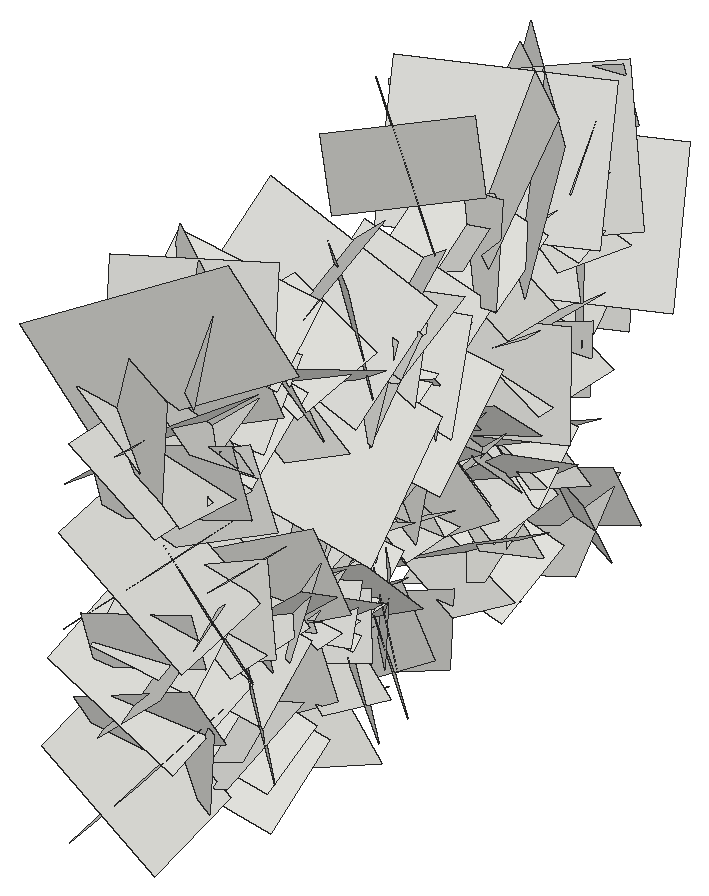
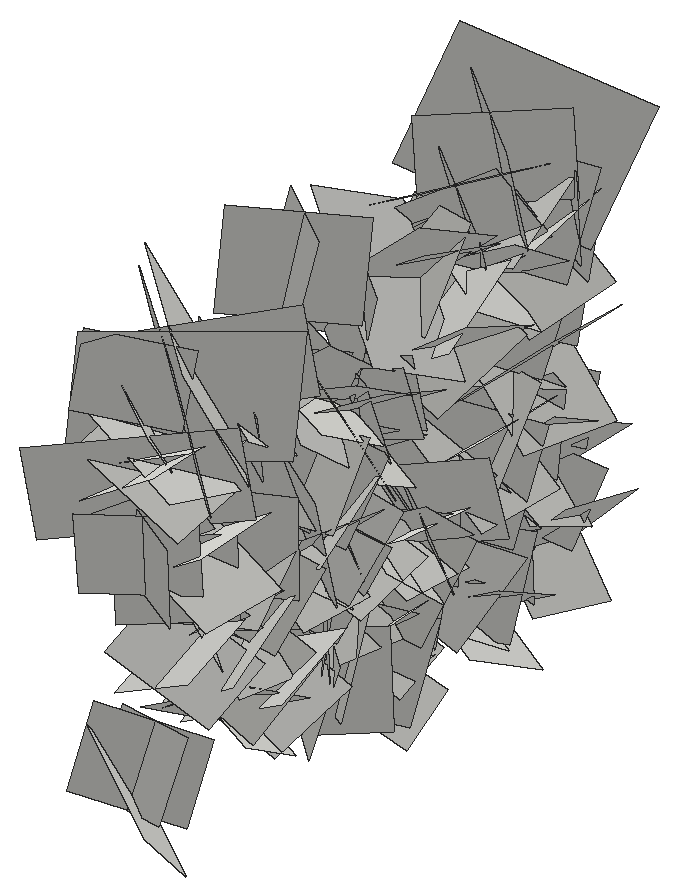
# SketchUp Ruby script. Lengths in inches.
U = 1.inch
M = Sketchup.active_model
def pt(a) = Geom::Point3d.new(a.map { |v| v * U })
def face(e, loops, mat)
  f = e.add_face(loops[0].map { |a| pt(a) })
  loops[1..].each { |l| e.add_face(l.map { |a| pt(a) }).erase! }
  f.material = f.back_material = mat if mat
  f
end
# faces: each face lists its corners as indices into pts; further lists are holes
def faces(e, pts, list, mat = nil) = list.each { |f| face(e, (f[0].is_a?(Array) ? f : [f]).map { |l| l.map { |i| pts[i] } }, mat) }
# xy, xz, yz: faces in a plane at the given z, y or x. An outline is a flat list of corners, or four numbers for a rectangle; further outlines are holes
def ring(l) = l.size == 4 ? [[l[0], l[1]], [l[2], l[1]], [l[2], l[3]], [l[0], l[3]]] : l.each_slice(2).to_a
def flat(e, list, mat, &to3) = list.each { |f| face(e, (f[0].is_a?(Array) ? f : [f]).map { |l| ring(l).map { |u, v| to3.(u, v) } }, mat) }
def xy(e, z, list, mat = nil) = flat(e, list, mat) { |x, y| [x, y, z] }
def xz(e, y, list, mat = nil) = flat(e, list, mat) { |x, z| [x, y, z] }
def yz(e, x, list, mat = nil) = flat(e, list, mat) { |y, z| [x, y, z] }
def lines(e, pts, list) = list.each { |a, b| e.add_line(pt(pts[a]), pt(pts[b])) }
# prism: a flat outline (further loops are holes) pulled along v
def prism(e, loops, v, mat = nil)
  f = face(e, loops, mat); d = Geom::Vector3d.new(v.map { |x| x * U })
  f.pushpull(f.normal.samedirection?(d) ? d.length : -d.length)
end
def box(e, o, s, mat = nil) = prism(e, [[o, [o[0] + s[0], o[1], o[2]], [o[0] + s[0], o[1] + s[1], o[2]], [o[0], o[1] + s[1], o[2]]]], [0, 0, s[2]], mat)
def at(x, y, z, deg = 0) = Geom::Transformation.translation(pt([x, y, z])) * Geom::Transformation.rotation(ORIGIN, Z_AXIS, deg.degrees)
def axes(o, x, y, z) = Geom::Transformation.new([*x, 0, *y, 0, *z, 0, *pt(o).to_a, 1])
def part(name) = M.definitions.add(name)
# library, detail: a bought-in or finely detailed component or shape, given as its bounding box
def library(name, o, s) = part(name).tap { |d| box(d.entities, o, s) }
def detail(e, o, s) = box(e.add_group.entities, o, s)
def put(e, d, t, mat = nil) = e.add_instance(d, t).tap { |i| i.material = mat if mat }
def group(e, t, mat = nil) = e.add_group.tap { |g| g.transformation = t; g.material = mat if mat }.entities
root = M.entities
c1 = part("Component\#6")
p = [[0.01,0,0],[0,3.24,4.54],[4.32,3.24,4.54],[4.33,0,0]]
faces(c1.entities,p,[[0,1,2,3]])
put(root,c1,axes([400.91,150.44,37.52],[-0.01758,-0.03984,-0.83316],[0.08726,-0.82933,0.03802],[0.87984,0.08145,-0.02042]))
put(root,c1,axes([404.88,150.81,32.67],[0.03105,-0.70657,0.01303],[-0.00041,0.01303,0.70717],[-0.74909,-0.02929,0.00015]))
put(root,c1,axes([404.88,149.71,29.1],[-0.04042,0.22115,-0.567],[-0.10046,-0.56334,-0.21335],[-0.63725,0.07479,0.0696]))
put(root,c1,axes([400.91,147.16,24.1],[-0.03025,0.92414,0.23442],[-0.23339,0.2218,-0.90118],[0.98329,0.08108,-0.20669]))
put(root,c1,axes([404.88,147.16,24.1],[0.03025,0.92414,0.23442],[0.23339,0.2218,-0.90118],[-0.98329,0.08108,-0.20669]))
put(root,c1,axes([404.88,149.63,26.39],[0.05575,0.3601,-0.58557],[-0.15834,-0.56726,-0.36226],[-0.71127,0.15451,0.03475]))
put(root,c1,axes([400.91,149.65,34.23],[-0.2234,-0.54463,1.08834],[-0.02633,1.10624,0.54877],[1.28976,-0.07175,0.19972]))
put(root,c1,axes([404.88,151.89,27.92],[-0.07457,-0.37507,-0.49968],[0.035,-0.50437,0.37394],[-0.66135,0.0156,0.07613]))
put(root,c1,axes([400.91,152.86,25.21],[0.07237,-0.84668,-0.40971],[-0.16913,-0.41526,0.83156],[0.98259,-0.00911,0.17331]))
put(root,c1,axes([404.88,152.86,25.21],[-0.07237,-0.84668,-0.40971],[0.16913,-0.41526,0.83156],[-0.98259,-0.00911,0.17331]))
put(root,c1,axes([400.91,153.18,27.99],[-0.08911,-1.01671,-0.11332],[-0.1646,-0.0997,1.00972],[1.07181,-0.09984,0.14565]))
put(root,c1,axes([404.88,153.18,27.99],[0.08911,-1.01671,-0.11332],[0.1646,-0.0997,1.00972],[-1.07181,-0.09984,0.14565]))
put(root,c1,axes([400.91,150.4,30.92],[0.04252,-0.27759,0.76161],[0.13298,0.75548,0.26875],[0.84891,-0.10444,-0.08025]))
put(root,c1,axes([400.91,152.86,32.22],[-0.07765,-0.95123,0.12327],[-0.10469,0.13045,0.94796],[1.01133,-0.05954,0.1076]))
put(root,c1,axes([404.88,152.86,32.22],[0.07765,-0.95123,0.12327],[0.10469,0.13045,0.94796],[-1.01133,-0.05954,0.1076]))
put(root,c1,axes([400.91,150.92,33.45],[-0.01124,-0.40239,0.85237],[0.02564,0.85203,0.40253],[0.99881,-0.0264,-0.00074]))
put(root,c1,axes([400.91,150.56,37.37],[0.01495,0.72639,-0.4873],[0.06872,-0.48689,-0.7239],[0.92463,0.02444,0.06168]))
put(root,c1,axes([404.88,150.69,21.46],[0.08617,-0.06424,0.73191],[-0.1147,0.7273,0.07585],[-0.77031,-0.11548,0.07058]))
put(root,c1,axes([404.88,152.7,33.94],[0.15183,0.13661,-0.74127],[-0.04087,-0.75222,-0.14607],[-0.79793,0.06452,-0.13357]))
put(root,c1,axes([404.88,153.52,29.46],[0.08102,0.00764,-0.81457],[0.10707,-0.81193,0.00187],[-0.85682,-0.10074,-0.07679]))
put(root,c1,axes([400.91,154.14,39.875],[-0.07687,-0.17009,-0.90128],[-0.07958,-0.89996,0.17589],[0.96896,-0.0874,-0.05706]))
put(root,c1,axes([404.88,154.14,39.875],[0.07687,-0.17009,-0.90128],[0.07958,-0.89996,0.17589],[-0.96896,-0.0874,-0.05706]))
put(root,c1,axes([400.91,152.27,30.34],[0.04267,0.47891,-0.74389],[0.05776,-0.74459,-0.47642],[0.93603,0.02411,0.06331]))
put(root,c1,axes([404.88,155.3,36.05],[0.02231,-0.46484,-0.62566],[0.10069,-0.6197,0.4636],[-0.82005,-0.08874,0.0399]))
put(root,c1,axes([404.88,155.63,34.51],[0.04715,-0.7148,-0.47013],[-0.06325,-0.47221,0.71232],[-0.90467,-0.00424,-0.0743]))
put(root,c1,axes([400.91,155.63,34.51],[-0.04715,-0.7148,-0.47013],[0.06325,-0.47221,0.71232],[0.90467,-0.00424,-0.0743]))
put(root,c1,axes([400.91,151.43,29.49],[-0.01376,0.93036,0.01045],[-0.09599,0.00914,-0.92605],[0.98156,0.01394,-0.09041]))
put(root,c1,axes([404.88,151.43,29.49],[0.01376,0.93036,0.01045],[0.09599,0.00914,-0.92605],[-0.98156,0.01394,-0.09041]))
put(root,c1,axes([404.88,156.34,37.48],[0.20366,-0.78098,-0.33642],[-0.07649,-0.35863,0.79133],[-0.89812,-0.14656,-0.14368]))
put(root,c1,axes([400.91,152.31,24.83],[0.14132,0.38772,0.61473],[0.11706,0.60692,-0.40674],[0.76145,-0.16526,-0.05156]))
put(root,c1,axes([400.91,152.23,36.27],[0.17612,0.33723,0.58016],[-0.03508,0.60107,-0.33991],[0.71045,-0.05392,-0.16061]))
put(root,c1,axes([404.88,152.23,36.27],[-0.17612,0.33723,0.58016],[0.03508,0.60107,-0.33991],[-0.71045,-0.05392,-0.16061]))
put(root,c1,axes([400.91,151.53,22],[-0.08087,0.78957,0.40941],[0.10212,0.41583,-0.78401],[0.93722,0.02282,0.12075]))
put(root,c1,axes([404.88,151.53,22],[0.08087,0.78957,0.40941],[-0.10212,0.41583,-0.78401],[-0.93722,0.02282,0.12075]))
put(root,c1,axes([404.88,153.82,25.23],[-0.04726,-0.11023,0.59197],[-0.093,0.58845,0.10297],[-0.63147,-0.07841,-0.05947]))
put(root,c1,axes([400.91,156.05,22.34],[0.04217,-0.56806,-0.37659],[0.07293,-0.37196,0.56834],[0.71876,0.07107,-0.03557]))
put(root,c1,axes([404.88,156.05,22.34],[-0.04217,-0.56806,-0.37659],[-0.07293,-0.37196,0.56834],[-0.71876,0.07107,-0.03557]))
put(root,c1,axes([400.91,153.79,24.7],[-0.00565,-0.43188,0.90191],[-0.04751,0.90112,0.43124],[1.05892,0.03812,0.02416]))
put(root,c1,axes([400.91,153.92,21.15],[-0.0271,-0.2919,0.8704],[-0.20523,0.85287,0.28034],[0.95124,0.17569,0.08528]))
put(root,c1,axes([404.88,153.92,21.15],[0.0271,-0.2919,0.8704],[0.20523,0.85287,0.28034],[-0.95124,0.17569,0.08528]))
put(root,c1,axes([400.91,156.72,22.08],[-0.00521,-0.94479,0.50901],[-0.17637,0.50353,0.93301],[1.12382,0.07464,0.14878]))
put(root,c1,axes([400.91,155.99,38.05],[0.0315,0.52335,-0.79271],[-0.01447,-0.79278,-0.52391],[1.00678,-0.02777,0.01727]))
put(root,c1,axes([404.88,157.73,31.39],[0.13129,-0.92283,0.37392],[-0.04334,0.37177,0.93107],[-1.05456,-0.13017,0.00829]))
put(root,c1,axes([400.91,157.73,31.39],[-0.13129,-0.92283,0.37392],[0.04334,0.37177,0.93107],[1.05456,-0.13017,0.00829]))
put(root,c1,axes([400.91,154.45,36.57],[0.07713,0.81709,0.22722],[0.03645,0.22503,-0.82021],[0.89825,-0.07929,0.01378]))
put(root,c1,axes([404.88,158.82,28.52],[0.0834,-0.34729,-0.88838],[-0.00654,-0.89156,0.34799],[-1.01106,-0.02288,-0.07553]))
put(root,c1,axes([400.91,158.82,28.52],[-0.0834,-0.34729,-0.88838],[0.00654,-0.89156,0.34799],[1.01106,-0.02288,-0.07553]))
put(root,c1,axes([404.88,158.01,30.39],[-0.08038,-0.60995,0.00551],[0.02253,0.00291,0.6143],[-0.64618,0.07598,0.02073]))
put(root,c1,axes([400.91,152.65,32.7],[-0.31384,1.21799,0.62272],[-0.13011,0.61092,-1.25326],[1.44417,0.31973,0.02242]))
put(root,c1,axes([404.88,158.73,27.09],[0.13155,-0.14233,-0.74779],[0.00006,-0.75766,0.14422],[-0.80689,-0.02326,-0.12191]))
put(root,c1,axes([404.88,156.02,27.27],[-0.01737,0.78195,0.05447],[-0.0729,0.05284,-0.77921],[-0.82768,-0.02106,0.06749]))
put(root,c1,axes([400.91,156.02,27.27],[0.01737,0.78195,0.05447],[0.0729,0.05284,-0.77921],[0.82768,-0.02106,0.06749]))
put(root,c1,axes([404.88,156.49,28.09],[-0.01227,0.36562,0.53928],[-0.0952,0.53332,-0.36351],[-0.68404,-0.08079,0.04092]))
put(root,c1,axes([400.91,158.65,23.12],[-0.03,-0.65446,0.65644],[0.11713,0.64968,0.65248],[0.97555,-0.09812,-0.05816]))
put(root,c1,axes([404.88,154.61,36.92],[0.07328,1.03426,0.55463],[0.26621,0.52968,-1.01904],[-1.21518,0.17841,-0.1898]))
put(root,c1,axes([400.91,154.61,36.92],[-0.07328,1.03426,0.55463],[-0.26621,0.52968,-1.01904],[1.21518,0.17841,-0.1898]))
put(root,c1,axes([404.88,160.42,26.72],[0.04031,-0.6417,-0.5437],[-0.04231,-0.54502,0.64047],[-0.89052,-0.00315,-0.05504]))
put(root,c1,axes([400.91,160.42,26.72],[-0.04031,-0.6417,-0.5437],[0.04231,-0.54502,0.64047],[0.89052,-0.00315,-0.05504]))
put(root,c1,axes([400.91,159.35,19.53],[0.12506,-0.65018,0.20227],[-0.00025,0.20525,0.65988],[0.72178,0.11273,-0.03482]))
put(root,c1,axes([404.88,159.35,19.53],[-0.12506,-0.65018,0.20227],[0.00025,0.20525,0.65988],[-0.72178,0.11273,-0.03482]))
put(root,c1,axes([400.91,159.76,21.63],[0.09665,-0.666,0.12875],[-0.03078,0.12595,0.67212],[0.71837,0.095,0.01147]))
put(root,c1,axes([404.88,159.76,21.63],[-0.09665,-0.666,0.12875],[0.03078,0.12595,0.67212],[-0.71837,0.095,0.01147]))
put(root,c1,axes([404.88,158.75,26.14],[-0.12859,0.59437,-0.23179],[0.06253,-0.22448,-0.60651],[-0.67335,-0.13435,-0.01206]))
put(root,c1,axes([400.91,160.84,30.26],[0.09118,-0.56201,-0.30691],[0.0596,-0.30185,0.56849],[0.67615,0.1024,-0.00872]))
put(root,c1,axes([404.88,160.84,30.26],[-0.09118,-0.56201,-0.30691],[-0.0596,-0.30185,0.56849],[-0.67615,0.1024,-0.00872]))
put(root,c1,axes([400.91,160.9375,37.33],[0.13153,0.12633,-0.90974],[-0.10231,-0.91113,-0.13969],[0.96819,-0.11344,0.10882]))
put(root,c1,axes([400.91,159.1875,20.3125],[-0.01409,-0.35632,0.80543],[-0.16766,0.79339,0.34838],[0.91839,0.13938,0.07596]))
put(root,c1,axes([404.88,159.1875,20.3125],[0.01409,-0.35632,0.80543],[0.16766,0.79339,0.34838],[-0.91839,0.13938,0.07596]))
put(root,c1,axes([404.88,161.57,34.4],[0.05292,-0.24359,-0.78611],[-0.1523,-0.77804,0.23197],[-0.85897,0.12294,-0.08956]))
put(root,c1,axes([400.91,161.57,34.4],[-0.05292,-0.24359,-0.78611],[0.1523,-0.77804,0.23197],[0.85897,0.12294,-0.08956]))
put(root,c1,axes([404.88,158.35,30.49],[0.08461,0.81055,-0.03501],[0.12527,-0.04642,-0.80528],[-0.85081,0.07377,-0.12204]))
put(root,c1,axes([400.91,161.79,25.53],[0.01152,-0.82607,0.19056],[0.15176,0.18963,0.81386],[0.88572,-0.02175,-0.14193]))
put(root,c1,axes([400.91,162.32,28.44],[0.12821,-0.42216,-0.69512],[-0.01339,-0.70366,0.42514],[0.86197,0.05186,0.11]))
put(root,c1,axes([404.88,158.39,26.84],[0.02686,0.84806,0.10272],[0.17857,0.09579,-0.83237],[-0.88773,0.04493,-0.16432]))
put(root,c1,axes([400.91,157.3125,32.29],[-0.25179,1.05256,0.51222],[0.06429,0.53303,-1.06718],[1.23914,0.18623,0.15945]))
put(root,c1,axes([404.88,158.45,30.92],[0.16236,0.46297,0.88251],[-0.09478,0.89566,-0.45434],[-1.05211,-0.00924,0.17712]))
put(root,c1,axes([400.91,158.45,30.92],[-0.16236,0.46297,0.88251],[0.09478,0.89566,-0.45434],[1.05211,-0.00924,0.17712]))
put(root,c1,axes([404.88,160.06,22.6],[0.02839,-0.24478,0.77995],[0.15528,0.76918,0.23637],[-0.85248,0.13195,0.06903]))
put(root,c1,axes([404.88,159.46,22.85],[0.09982,-0.0635,0.89488],[0.1784,0.88507,0.04509],[-0.93408,0.16225,0.10424]))
put(root,c1,axes([404.88,162.92,24.26],[-0.16568,0.16434,-0.80239],[0.1251,-0.80382,-0.18763],[-0.85913,-0.14874,0.12742]))
put(root,c1,axes([400.91,162.92,24.26],[0.16568,0.16434,-0.80239],[-0.1251,-0.80382,-0.18763],[0.85913,-0.14874,0.12742]))
put(root,c1,axes([404.88,163.85,33.45],[0.03445,-0.73428,-0.4148],[-0.17499,-0.41262,0.71747],[-0.87664,0.05351,-0.15952]))
put(root,c1,axes([400.91,163.85,33.45],[-0.03445,-0.73428,-0.4148],[0.17499,-0.41262,0.71747],[0.87664,0.05351,-0.15952]))
put(root,c1,axes([404.88,162.43,26.35],[-0.02315,-0.70596,0.51236],[0.01203,0.51225,0.70629],[-0.92456,0.02434,-0.00364]))
put(root,c1,axes([400.91,162.43,26.35],[0.02315,-0.70596,0.51236],[-0.01203,0.51225,0.70629],[0.92456,0.02434,-0.00364]))
put(root,c1,axes([404.88,162.61,28.57],[0.04222,-0.49534,0.62953],[-0.20196,0.60636,0.48917],[-0.82474,-0.17384,-0.08755]))
put(root,c1,axes([400.91,162.61,28.57],[-0.04222,-0.49534,0.62953],[0.20196,0.60636,0.48917],[0.82474,-0.17384,-0.08755]))
put(root,c1,axes([404.88,162.33,29.83],[0.22776,0.38392,-0.75072],[-0.01782,-0.77261,-0.39993],[-0.89361,0.11326,-0.18337]))
put(root,c1,axes([400.91,164.2,31.01],[-0.06613,-0.18181,-0.96198],[0.02897,-0.96387,0.1804],[1.03734,0.01533,-0.06637]))
put(root,c1,axes([404.88,159.67,28.14],[0.12868,0.67272,0.52517],[0.08613,0.51893,-0.68352],[-0.90053,0.14576,0.00967]))
put(root,c1,axes([400.91,164.96,33.58],[0.03363,-0.67551,-0.53197],[-0.14584,-0.52946,0.66412],[0.89967,-0.06058,0.12754]))
put(root,c1,axes([404.88,164.96,33.58],[-0.03363,-0.67551,-0.53197],[0.14584,-0.52946,0.66412],[-0.89967,-0.06058,0.12754]))
put(root,c1,axes([404.88,164.8,26.41],[-0.06555,-0.88967,-0.10275],[0.1194,-0.1099,0.88381],[-0.94178,0.04799,0.1192]))
put(root,c1,axes([400.91,164.8,26.41],[0.06555,-0.88967,-0.10275],[-0.1194,-0.1099,0.88381],[0.94178,0.04799,0.1192]))
put(root,c1,axes([404.88,163.99,40.83],[-0.08038,0.23372,-0.81219],[0.10222,-0.80774,-0.24144],[-0.89001,-0.11388,0.04562]))
put(root,c1,axes([400.91,163.99,40.83],[0.08038,0.23372,-0.81219],[-0.10222,-0.80774,-0.24144],[0.89001,-0.11388,0.04562]))
put(root,c1,axes([404.88,166.33,22.3],[0.05809,-0.87115,0.26873],[-0.09257,0.26296,0.87026],[-0.96191,-0.07791,-0.06752]))
put(root,c1,axes([400.91,166.33,22.3],[-0.05809,-0.87115,0.26873],[0.09257,0.26296,0.87026],[0.96191,-0.07791,-0.06752]))
put(root,c1,axes([404.88,164.95,29.96],[0.04265,0.57286,-0.52342],[-0.15347,-0.50938,-0.56862],[-0.80809,0.12697,0.08036]))
put(root,c1,axes([400.91,164.95,29.96],[-0.04265,0.57286,-0.52342],[0.15347,-0.50938,-0.56862],[0.80809,0.12697,0.08036]))
put(root,c1,axes([400.91,167.29,35.58],[0.17595,-0.29467,-0.74084],[0.05215,-0.7515,0.30993],[0.84352,0.10793,0.13537]))
put(root,c1,axes([400.91,167.69,34.89],[0.01272,-0.59445,-0.3878],[0.01652,-0.38754,0.59453],[0.75216,0.01856,-0.0065]))
put(root,c1,axes([404.88,167.69,34.89],[-0.01272,-0.59445,-0.3878],[-0.01652,-0.38754,0.59453],[-0.75216,0.01856,-0.0065]))
put(root,c1,axes([400.91,168.18,25.35],[0.0356,-0.79141,-0.13903],[-0.13499,-0.14264,0.78117],[0.84098,0.01061,0.13127]))
put(root,c1,axes([404.88,168.18,25.35],[-0.0356,-0.79141,-0.13903],[0.13499,-0.14264,0.78117],[-0.84098,0.01061,0.13127]))
put(root,c1,axes([404.88,164.5,23.79],[-0.04443,0.667,0.37408],[-0.11412,0.36576,-0.66423],[-0.80255,-0.08894,0.07374]))
put(root,c1,axes([400.91,164.5,23.79],[0.04443,0.667,0.37408],[0.11412,0.36576,-0.66423],[0.80255,-0.08894,0.07374]))
put(root,c1,axes([400.91,165.04,27.71],[-0.04822,0.07219,0.94774],[0.14201,0.93984,-0.06516],[0.99746,-0.13032,0.05509]))
put(root,c1,axes([404.88,167.51,23.32],[0.04127,-0.8056,0.43064],[0.05085,0.43224,0.80425],[-0.96695,-0.01165,0.06068]))
put(root,c1,axes([400.91,167.51,23.32],[-0.04127,-0.8056,0.43064],[-0.05085,0.43224,0.80425],[0.96695,-0.01165,0.06068]))
put(root,c1,axes([404.88,168.23,31.98],[0.11552,-0.73847,0.10601],[-0.00435,0.10653,0.74638],[-0.79079,-0.10846,0.01138]))
put(root,c1,axes([404.88,169.17,27.35],[-0.00515,-0.4485,-0.48712],[-0.04455,-0.48594,0.44784],[-0.70046,0.0342,-0.02491]))
put(root,c1,axes([404.88,171.21,38.93],[0.24063,-0.51313,-1.11059],[0.16085,-1.10901,0.54342],[-1.28679,-0.23458,-0.13976]))
put(root,c1,axes([400.91,171.21,38.93],[-0.24063,-0.51313,-1.11059],[-0.16085,-1.10901,0.54342],[1.28679,-0.23458,-0.13976]))
put(root,c1,axes([404.88,166.53,31.68],[0.02185,0.89564,-0.0065],[-0.05171,-0.00537,-0.89456],[-0.948,0.02094,0.04865]))
put(root,c1,axes([400.91,166.53,31.68],[-0.02185,0.89564,-0.0065],[0.05171,-0.00537,-0.89456],[0.948,0.02094,0.04865]))
put(root,c1,axes([400.91,169.82,24.93],[0.00586,-0.68753,0.27068],[0.05817,0.27032,0.6855],[0.78107,-0.01497,-0.05308]))
put(root,c1,axes([404.88,169.82,24.93],[-0.00586,-0.68753,0.27068],[-0.05817,0.27032,0.6855],[-0.78107,-0.01497,-0.05308]))
put(root,c1,axes([404.88,169.92,30.86],[-0.08798,0.07784,-0.70174],[0.08853,-0.70052,-0.08758],[-0.74315,-0.09267,0.07264]))
put(root,c1,axes([404.88,171.77,39.47],[0.25632,-0.1505,-1.28885],[0.2021,-1.29268,0.18672],[-1.36053,-0.22038,-0.21508]))
put(root,c1,axes([400.91,171.77,39.47],[-0.25632,-0.1505,-1.28885],[-0.2021,-1.29268,0.18672],[1.36053,-0.22038,-0.21508]))
put(root,c1,axes([400.91,171.89,34.33],[-0.10287,-0.74562,-0.1631],[0.15609,-0.17961,0.73351],[0.79385,-0.06131,-0.16536]))
put(root,c1,axes([404.88,171.89,34.33],[0.10287,-0.74562,-0.1631],[-0.15609,-0.17961,0.73351],[-0.79385,-0.06131,-0.16536]))
put(root,c1,axes([404.88,171.91,32.4],[-0.07209,-0.36069,-0.54144],[0.07785,-0.54516,0.35394],[-0.6852,-0.024,0.09718]))
put(root,c1,axes([404.88,168.875,35.8],[-0.07444,0.7996,-0.0855],[-0.00091,-0.0859,-0.80263],[-0.85241,-0.06974,0.00832]))
put(root,c1,axes([400.91,168.875,35.8],[0.07444,0.7996,-0.0855],[0.00091,-0.0859,-0.80263],[0.85241,-0.06974,0.00832]))
put(root,c1,axes([404.88,168.82,35.84],[-0.04533,0.37689,0.51175],[0.01637,0.51337,-0.3768],[-0.67349,-0.01289,-0.04361]))
put(root,c1,axes([400.91,167.34,31.77],[-0.2501,0.51374,1.1242],[-0.05799,1.13903,-0.532],[1.3089,0.14863,0.19123]))
put(root,c1,axes([400.91,172.01,32.68],[0.01531,-0.04852,-0.71126],[0.05574,-0.70939,0.04946],[0.75363,0.05345,0.01079]))
put(root,c1,axes([404.88,172.01,32.68],[-0.01531,-0.04852,-0.71126],[-0.05574,-0.70939,0.04946],[-0.75363,0.05345,0.01079]))
put(root,c1,axes([400.91,170.91,25.11],[0.00896,0.33986,-0.6335],[0.15678,-0.62081,-0.33108],[0.74574,0.12644,0.07722]))
put(root,c1,axes([404.88,170.91,25.11],[-0.00896,0.33986,-0.6335],[-0.15678,-0.62081,-0.33108],[-0.74574,0.12644,0.07722]))
put(root,c1,axes([404.88,171.42,39.46],[-0.01769,0.21401,-0.61924],[-0.03571,-0.6189,-0.21298],[-0.69357,0.02641,0.02676]))
put(root,c1,axes([404.88,169.05,21.98],[-0.04882,0.58162,0.59704],[0.02934,0.59868,-0.58109],[-0.88303,-0.01226,-0.05232]))
